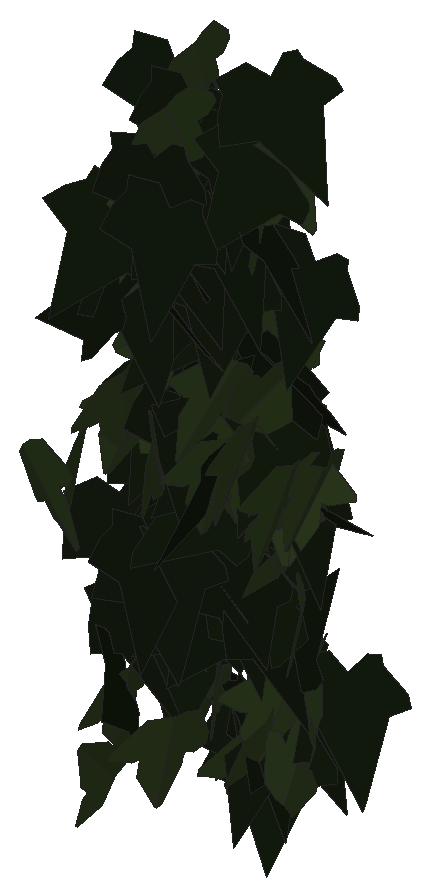
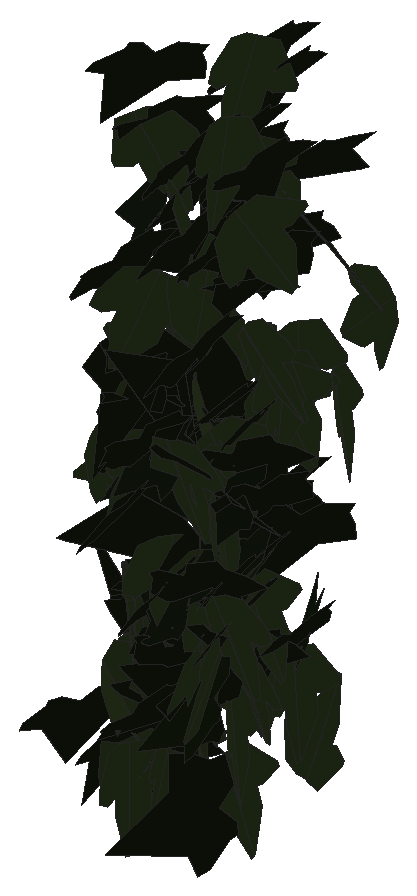
# SketchUp Ruby script. Lengths in inches.
U = 1.inch
M = Sketchup.active_model
def pt(a) = Geom::Point3d.new(a.map { |v| v * U })
def face(e, loops, mat)
  f = e.add_face(loops[0].map { |a| pt(a) })
  loops[1..].each { |l| e.add_face(l.map { |a| pt(a) }).erase! }
  f.material = f.back_material = mat if mat
  f
end
# faces: each face lists its corners as indices into pts; further lists are holes
def faces(e, pts, list, mat = nil) = list.each { |f| face(e, (f[0].is_a?(Array) ? f : [f]).map { |l| l.map { |i| pts[i] } }, mat) }
# xy, xz, yz: faces in a plane at the given z, y or x. An outline is a flat list of corners, or four numbers for a rectangle; further outlines are holes
def ring(l) = l.size == 4 ? [[l[0], l[1]], [l[2], l[1]], [l[2], l[3]], [l[0], l[3]]] : l.each_slice(2).to_a
def flat(e, list, mat, &to3) = list.each { |f| face(e, (f[0].is_a?(Array) ? f : [f]).map { |l| ring(l).map { |u, v| to3.(u, v) } }, mat) }
def xy(e, z, list, mat = nil) = flat(e, list, mat) { |x, y| [x, y, z] }
def xz(e, y, list, mat = nil) = flat(e, list, mat) { |x, z| [x, y, z] }
def yz(e, x, list, mat = nil) = flat(e, list, mat) { |y, z| [x, y, z] }
def lines(e, pts, list) = list.each { |a, b| e.add_line(pt(pts[a]), pt(pts[b])) }
# prism: a flat outline (further loops are holes) pulled along v
def prism(e, loops, v, mat = nil)
  f = face(e, loops, mat); d = Geom::Vector3d.new(v.map { |x| x * U })
  f.pushpull(f.normal.samedirection?(d) ? d.length : -d.length)
end
def box(e, o, s, mat = nil) = prism(e, [[o, [o[0] + s[0], o[1], o[2]], [o[0] + s[0], o[1] + s[1], o[2]], [o[0], o[1] + s[1], o[2]]]], [0, 0, s[2]], mat)
def at(x, y, z, deg = 0) = Geom::Transformation.translation(pt([x, y, z])) * Geom::Transformation.rotation(ORIGIN, Z_AXIS, deg.degrees)
def axes(o, x, y, z) = Geom::Transformation.new([*x, 0, *y, 0, *z, 0, *pt(o).to_a, 1])
def part(name) = M.definitions.add(name)
# library, detail: a bought-in or finely detailed component or shape, given as its bounding box
def library(name, o, s) = part(name).tap { |d| box(d.entities, o, s) }
def detail(e, o, s) = box(e.add_group.entities, o, s)
def put(e, d, t, mat = nil) = e.add_instance(d, t).tap { |i| i.material = mat if mat }
def group(e, t, mat = nil) = e.add_group.tap { |g| g.transformation = t; g.material = mat if mat }.entities
root = M.entities
M.materials.add("efeu1").color = [18, 25, 13]
M.materials.add("efeu2").color = [43, 57, 29]
c1 = part("ivyleaf_10")
p = [[0,0.5,-0.03],[-0.0625,2.02,-0.43],[-0.19,2.01,-0.46],[-0.54,1.05,-0.29],[-0.52,0.625,-0.18],[-0.83,0.76,-0.28],
  [-1.16,0.64,-0.33],[-1.15,0.33,-0.24],[-0.77,-0.39,0.02],[-0.3,-0.51,0.16],[0.04,-0.48,0.23],[-0.02,2.01,-0.4375],
  [-0.06,2.01,-0.43],[0.04,-0.49,0.23],[0.67,-0.49,0.14],[1.38,0.36,-0.2],[1.375,0.51,-0.24],[0.81,0.65,-0.19],
  [0.62,0.59,-0.15],[0.6,1.09,-0.28],[0.5,1.23,-0.31]]
faces(c1.entities,p,[[0,1,2,3,4,5,6,7,8,9,10],[11,12,0,13,14,15,16,17,18,19,20]],"efeu2")
c2 = part("ivyleaf_9")
p = [[1.54,2.16,1.25],[1.36,2.04,1.19],[-0.21,0.99,0.68],[-0.71,1.11,0.82],[-0.85,0.86,0.67],[-0.8,0.17,0.21],
  [-0.9,-0.01,0.1],[-0.67,-0.16,-0.02],[-0.08,-0.08,-0.05],[-0.03,-0.6,-0.4],[0.65,-0.88,-0.66],[0.83,-0.6,-0.49],
  [1.29,-0.42,-0.43],[1.8125,-0.07,-0.26],[1.21,0.44,0.15]]
faces(c2.entities,p,[[0,1,2,3,4,5,6,7,8,9,10,11,12,13,14]],"efeu1")
put(root,c1,axes([21.42,223.09,234.66],[0.162,-0.45556,-0.12737],[-0.01354,0.13011,-0.48258],[0.47284,0.1598,0.02982]))
put(root,c1,axes([21.47,223.21,235.97],[0.45383,-0.08336,-0.19259],[-0.1748,0.10376,-0.45681],[0.11612,0.48196,0.06503]))
put(root,c1,axes([21.52,222.74,240.73],[-0.16134,-0.38229,0.27896],[-0.05629,-0.27714,-0.41234],[0.46989,-0.16446,0.04639]))
put(root,c1,axes([21.4,222.91,235.22],[0.44303,-0.23126,-0.0156],[-0.01307,0.00866,-0.49975],[0.23141,0.44322,0.00163]))
put(root,c1,axes([21.46,221.16,237.97],[0.20397,-0.44652,-0.09496],[-0.01699,0.09651,-0.4903],[0.45619,0.20324,0.02419]))
put(root,c2,axes([21.33,222.99,241.68],[-0.10782,-0.48667,0.03903],[-0.0065,-0.03854,-0.49847],[0.48819,-0.10799,0.00199]))
put(root,c1,axes([21.48,222.62,235.85],[0.05393,-0.48608,0.10401],[0.00285,-0.10432,-0.48899],[0.49708,0.05333,-0.00848]))
put(root,c1,axes([21.42,221.75,233.52],[-0.04473,-0.33215,-0.37105],[-0.02937,-0.37013,0.33487],[-0.49713,0.05175,0.0136]))
put(root,c1,axes([21.51,221.875,234.64],[-0.00249,-0.49392,-0.07773],[0.01152,0.07765,-0.4938],[0.49986,-0.00425,0.011]))
put(root,c1,axes([21.52,223.01,233.81],[0.02957,-0.4962,0.05394],[-0.00482,-0.05432,-0.49702],[0.4991,0.02887,-0.00799]))
put(root,c1,axes([21.7,222.32,238.99],[0.3077,-0.16583,-0.35752],[-0.32173,0.15627,-0.34938],[0.22762,0.44506,-0.01054]))
put(root,c2,axes([21.26,222.3,235.39],[0.1524,-0.45433,-0.14269],[-0.00329,0.14882,-0.47733],[0.4762,0.14643,0.04237]))
put(root,c2,axes([21.54,222.94,237.9],[-0.3472,-0.35905,-0.02316],[0.01678,0.01599,-0.49946],[0.3594,-0.3476,0.00095]))
put(root,c2,axes([21.33,222.05,236.78],[-0.05664,-0.4023,-0.29145],[0.09276,0.27962,-0.40399],[0.48804,-0.09984,0.04296]))
put(root,c1,axes([21.54,223.25,235.35],[0.06205,-0.30518,-0.39118],[0.02748,0.39573,-0.30437],[0.49537,0.01627,0.06588]))
put(root,c1,axes([21.69,221.99,238.2],[-0.16252,-0.43116,0.19414],[-0.05936,-0.18505,-0.46069],[0.46911,-0.17279,0.00896]))
put(root,c2,axes([21.39,222.72,237.39],[0.00068,-0.44657,-0.2249],[0.06698,0.22295,-0.4425],[0.49549,-0.02953,0.06012]))
put(root,c1,axes([21.6,223.01,241.97],[-0.04509,-0.46727,-0.17213],[0.06125,0.16631,-0.46753],[0.49418,-0.06325,0.04224]))
put(root,c2,axes([21.26,223.68,233.76],[0.46894,-0.04796,0.16672],[0.16587,-0.0168,-0.47138],[0.05082,0.49741,0.00015]))
put(root,c1,axes([21.63,221.93,238.46],[-0.0639,-0.47515,-0.14196],[0.03474,0.13849,-0.47918],[0.49468,-0.0711,0.01532]))
put(root,c2,axes([21.75,223.53,236.5],[-0.4103,-0.28437,-0.02805],[0.02085,0.01915,-0.4992],[0.28499,-0.41081,-0.00386]))
put(root,c2,axes([21.45,222.77,236.49],[0.279,-0.33817,-0.24042],[-0.03835,0.26746,-0.42071],[0.41314,0.25319,0.1233]))
put(root,c2,axes([21.48,223.03,235.84],[0.11319,-0.48436,0.05084],[0.01191,-0.04943,-0.49741],[0.48687,0.11382,0.00035]))
put(root,c1,axes([21.77,223.03,235.92],[-0.08785,-0.49191,-0.01746],[0.00569,0.01672,-0.49969],[0.49219,-0.08799,0.00266]))
put(root,c2,axes([21.43,223.52,235.05],[0.41223,-0.28063,0.03616],[0.02669,-0.02504,-0.49866],[0.28169,0.41306,-0.00567]))
put(root,c1,axes([21.78,221.48,238.6],[-0.06652,-0.48285,-0.11149],[0.0163,0.1103,-0.48741],[0.49529,-0.06848,0.00106]))
put(root,c1,axes([21.79,222.87,237.08],[0.13997,-0.4719,-0.08784],[-0.01744,0.08644,-0.49216],[0.47969,0.14084,0.00774]))
put(root,c1,axes([21.82,222.875,237.83],[-0.12017,-0.44529,0.19308],[-0.02103,-0.19395,-0.46037],[0.48489,-0.11876,0.02788]))
put(root,c2,axes([22.1,221.02,239.98],[-0.36896,0.29037,0.17192],[-0.14342,0.09564,-0.46934],[-0.30545,-0.39565,0.01272]))
put(root,c2,axes([21.58,223.08,235.98],[0.04576,-0.44794,0.21739],[0.05491,-0.21244,-0.44928],[0.49486,0.06499,0.02975]))
put(root,c1,axes([21.68,222.75,237.7],[0.31352,0.38523,0.05747],[0.03252,0.04762,-0.49666],[-0.38813,0.31517,0.00481]))
put(root,c2,axes([21.63,221.74,234.6875],[-0.0113,-0.18597,0.46399],[0.03554,-0.46323,-0.1848],[0.49861,0.02881,0.02369]))
put(root,c1,axes([21.8,223.31,235.375],[-0.09842,0.45616,-0.17954],[-0.01552,-0.18593,-0.46389],[-0.48997,-0.08574,0.05075]))
put(root,c2,axes([21.8,222.66,235.18],[-0.22963,-0.42092,-0.14176],[0.05633,0.13069,-0.47932],[0.44056,-0.2361,-0.0126]))
put(root,c2,axes([21.93,221.29,240.81],[-0.2595,-0.39055,0.17357],[-0.03458,-0.18322,-0.46394],[0.42598,-0.25279,0.06808]))
put(root,c2,axes([21.8125,222.875,237.8],[-0.05662,-0.43271,0.24404],[-0.01462,-0.24406,-0.43614],[0.49657,-0.05653,0.01498]))
put(root,c2,axes([21.53,222.89,237.39],[0.36789,-0.17911,0.28736],[0.28472,-0.06605,-0.40568],[0.18329,0.46212,0.05339]))
put(root,c2,axes([21.59,222.74,236.25],[0.31209,-0.31312,0.23357],[0.16264,-0.16767,-0.44208],[0.35517,0.35192,-0.0028]))
put(root,c2,axes([22.28,223.18,237.62],[-0.4651,0.1003,0.1537],[-0.16048,-0.01909,-0.47316],[-0.08905,-0.48946,0.04995]))
put(root,c2,axes([21.54,223.33,234.87],[0.26945,-0.16012,0.38956],[0.34176,-0.18717,-0.31332],[0.24617,0.43512,0.00857]))
put(root,c2,axes([22.05,223.44,235.54],[-0.39421,-0.30689,-0.02043],[0.02036,0.0071,-0.49953],[0.3069,-0.39467,0.0069]))
put(root,c1,axes([22.06,223.32,237.83],[0.46354,-0.10321,-0.15646],[-0.14039,0.08538,-0.47223],[0.12419,0.48172,0.05018]))
put(root,c2,axes([21.81,222.45,238.43],[0.26422,-0.3478,-0.24336],[-0.02053,0.27584,-0.41652],[0.42399,0.2301,0.13148]))
put(root,c2,axes([21.9,222.57,241.67],[-0.0097,-0.49632,0.05973],[0.00706,-0.05987,-0.49635],[0.49986,-0.00878,0.00817]))
put(root,c2,axes([21.92,221.9,239.99],[0.04285,-0.36339,-0.34075],[0.01933,0.34297,-0.36332],[0.49779,0.01796,0.04344]))
put(root,c1,axes([21.95,223.07,234.23],[0.24182,-0.33251,0.28454],[0.22902,-0.18087,-0.406],[0.37293,0.32668,0.06483]))
put(root,c2,axes([22.33,222.28,237.85],[-0.41943,0.25092,-0.10543],[0.08583,-0.06185,-0.48868],[-0.25828,-0.42803,0.00881]))
put(root,c1,axes([22.18,222.15,235.93],[0.03203,-0.4986,0.0194],[-0.00168,-0.01955,-0.49961],[0.49897,0.03194,-0.00292]))
put(root,c1,axes([21.92,219.87,238.37],[-0.31494,0.19918,-0.33337],[0.27708,-0.18548,-0.37259],[-0.27209,-0.41943,0.00645]))
put(root,c1,axes([22.2,223.27,236.48],[-0.31951,-0.38451,-0.00816],[0.01625,-0.0029,-0.49973],[0.38426,-0.3196,0.01435]))
put(root,c2,axes([22.04,221.65,240.02],[-0.11955,-0.4542,-0.17148],[0.05718,0.1622,-0.46949],[0.48212,-0.13187,0.01316]))
put(root,c1,axes([21.97,222.98,234.72],[0.20651,-0.23119,0.3923],[0.289,-0.26635,-0.30909],[0.3519,0.35441,0.02362]))
put(root,c2,axes([22.37,223.03,235.51],[-0.01547,-0.09452,-0.49074],[-0.05993,-0.48708,0.0957],[-0.49615,0.06178,0.00374]))
put(root,c2,axes([22.01,223.15,239.18],[0.06323,-0.49592,0.00777],[0.00002,-0.00783,-0.49994],[0.49599,0.06323,-0.00098]))
put(root,c1,axes([22.34,221.69,240.8],[-0.29747,-0.27255,0.29534],[-0.06766,-0.32823,-0.37106],[0.39615,-0.26073,0.1584]))
put(root,c2,axes([22.07,222.19,238.1],[0.02234,-0.49726,0.04722],[0.01219,-0.04671,-0.49766],[0.49935,0.02339,0.01004]))
put(root,c2,axes([21.875,223.41,236.09],[0.1938,-0.3143,0.33713],[0.25838,-0.22877,-0.36181],[0.38168,0.31445,0.07375]))
put(root,c2,axes([22.11,221.62,236.62],[-0.027,-0.49436,0.06986],[0.00566,-0.07026,-0.49501],[0.49924,-0.02594,0.00939]))
put(root,c1,axes([22.28,222.56,238.28],[0.18808,-0.4428,0.13623],[0.03591,-0.13265,-0.48074],[0.46188,0.19062,-0.0181]))
put(root,c2,axes([22.36,222.23,239.5],[-0.32719,-0.33596,0.17342],[-0.03203,-0.20389,-0.45541],[0.37672,-0.30912,0.11191]))
put(root,c2,axes([22.32,222.68,237.5],[-0.23483,-0.32717,0.29634],[-0.04741,-0.31502,-0.38537],[0.43887,-0.20909,0.11693]))
put(root,c2,axes([22.21,221.67,236.59],[-0.16636,-0.40324,-0.24438],[0.09809,0.22387,-0.43619],[0.4612,-0.19307,0.00462]))
put(root,c1,axes([22.41,221.54,234.47],[-0.16861,-0.46925,0.03704],[-0.00513,-0.03752,-0.49856],[0.47068,-0.16851,0.00784]))
put(root,c1,axes([22.33,222.625,237.33],[0.38143,-0.32307,0.01158],[0.00448,-0.01262,-0.49982],[0.32325,0.3814,-0.00673]))
put(root,c2,axes([22.2,223.04,240.55],[0.02159,-0.49932,0.01473],[0.00105,-0.0147,-0.49978],[0.49953,0.02161,0.00041]))
put(root,c2,axes([22.52,222.46,237.01],[-0.40354,-0.2211,0.19563],[-0.08536,-0.2298,-0.43578],[0.28261,-0.38511,0.14772]))
put(root,c2,axes([22.29,222.51,235.57],[-0.11579,-0.37438,0.31053],[-0.00772,-0.31775,-0.38597],[0.48635,-0.09417,0.0678]))
put(root,c2,axes([22.22,223.46,236.12],[0.01098,-0.48222,0.13171],[0.01839,-0.13126,-0.48211],[0.49954,0.01544,0.01485]))
put(root,c2,axes([22.32,222.46,240.03],[-0.09351,-0.44748,0.20254],[-0.0305,-0.20049,-0.45703],[0.49023,-0.09783,0.0102]))
put(root,c1,axes([22.4,223.02,233.875],[0.07984,-0.44422,-0.21515],[0.07986,0.22671,-0.43844],[0.48708,0.03565,0.10715]))
put(root,c1,axes([22.41,221.56,242.11],[-0.15354,-0.42667,-0.21066],[0.09556,0.18919,-0.45285],[0.46615,-0.17932,0.02345]))
put(root,c2,axes([22.12,221.99,239.96],[0.05661,-0.18017,0.46296],[0.24382,-0.3959,-0.18389],[0.43284,0.24658,0.04304]))
put(root,c1,axes([22.47,221.14,238.18],[0.22506,-0.35692,-0.26825],[-0.01341,0.29487,-0.40358],[0.44628,0.18885,0.12315]))
put(root,c1,axes([22.33,222.29,237.83],[-0.43066,0.14503,-0.20857],[0.17682,-0.12363,-0.45105],[-0.18241,-0.46226,0.0552]))
put(root,c2,axes([22.375,223.71,234.62],[-0.14768,-0.45278,0.15225],[0.00242,-0.16006,-0.47368],[0.47769,-0.13917,0.04947]))
put(root,c2,axes([22.17,222.59,238.04],[0.05966,-0.10767,0.48461],[0.47529,0.15329,-0.02445],[-0.14331,0.46358,0.12064]))
put(root,c1,axes([22.4,222.59,239.15],[-0.03542,-0.36064,-0.34451],[0.03239,-0.34631,0.35919],[-0.49769,0.00313,0.0479]))
put(root,c1,axes([22.6,223.5,233.77],[-0.06793,-0.48401,-0.10543],[0.01343,0.10458,-0.48876],[0.49518,-0.06923,-0.0012]))
put(root,c2,axes([22.42,221.27,241.68],[0.00056,-0.49968,-0.01774],[0.00323,0.01774,-0.49967],[0.49999,0.00045,0.00325]))
put(root,c2,axes([22.32,222.96,237.89],[0.45104,-0.21578,0.00117],[0.00104,-0.00053,-0.5],[0.21578,0.45104,-0.00003]))
put(root,c1,axes([22.69,222.77,233.83],[-0.20021,-0.45679,0.03543],[-0.00656,-0.03581,-0.49867],[0.45812,-0.20014,0.00834]))
put(root,c2,axes([22.49,222.66,241.32],[0.00436,-0.49268,0.08515],[0.00196,-0.08513,-0.4927],[0.49998,0.00463,0.00119]))
put(root,c2,axes([22.42,223.25,233.88],[0.13552,-0.46598,0.12038],[0.02819,-0.11716,-0.48526],[0.48046,0.13831,-0.00549]))
put(root,c2,axes([22.98,222.93,235.625],[-0.41003,-0.01845,0.28555],[-0.24723,-0.22838,-0.36976],[0.14407,-0.44441,0.17816]))
put(root,c2,axes([22.3125,223.02,236.86],[0.42334,-0.05675,0.25992],[0.26398,0.02889,-0.42365],[0.03306,0.49593,0.05443]))
put(root,c1,axes([22.75,223.47,233.99],[0.01329,-0.49693,-0.05366],[0.00313,0.05376,-0.49709],[0.49981,0.01288,0.00454]))
put(root,c2,axes([22.69,223.18,237.8125],[-0.21508,-0.44975,0.03821],[-0.01308,-0.03609,-0.49852],[0.45119,-0.21545,0.00376]))
put(root,c2,axes([22.58,221.57,240.88],[0.03873,-0.44296,-0.22867],[-0.0182,0.22795,-0.44465],[0.49817,0.04277,0.00153]))
put(root,c2,axes([22.53,223,233.96],[0.01206,-0.31777,0.38585],[0.08535,-0.37898,-0.31478],[0.49251,0.07346,0.04511]))
put(root,c1,axes([22.76,222.91,236.0625],[-0.00585,-0.46562,-0.18211],[0.03678,0.18123,-0.46455],[0.49861,-0.01884,0.03213]))
put(root,c2,axes([22.99,222.78,238.69],[0.16494,0.10145,-0.46098],[-0.38257,-0.25728,-0.19351],[-0.27646,0.41655,-0.00725]))
put(root,c2,axes([22.59,222.54,236.14],[0.05196,-0.48821,-0.09459],[-0.00709,0.09437,-0.49096],[0.49724,0.05236,0.00288]))
put(root,c1,axes([22.85,221.93,238.84],[-0.07036,-0.4031,0.28734],[-0.00575,-0.28954,-0.40759],[0.49499,-0.06066,0.03611]))
put(root,c2,axes([22.72,222.14,240.13],[-0.17256,-0.46099,-0.08783],[0.02149,0.08572,-0.49213],[0.46879,-0.17362,-0.00977]))
put(root,c2,axes([22.73,223.04,233.81],[-0.22931,-0.4162,-0.15556],[0.06556,0.14144,-0.47507],[0.43945,-0.23827,-0.0103]))
put(root,c1,axes([22.89,221.8125,237.97],[-0.12038,-0.48031,0.06937],[0.00492,-0.07267,-0.49467],[0.48527,-0.11841,0.02223]))
put(root,c2,axes([22.66,223.43,234.24],[0.12808,-0.42708,-0.22627],[-0.03906,0.22417,-0.44522],[0.48174,0.13172,0.02406]))
put(root,c1,axes([22.87,222.42,240.62],[0.36772,-0.33729,-0.03191],[-0.02365,0.02142,-0.49898],[0.33797,0.36848,-0.0002]))
put(root,c2,axes([22.875,221.97,237.81],[-0.17867,0.00887,-0.4669],[0.30861,-0.37295,-0.12517],[-0.35048,-0.33291,0.12779]))
put(root,c2,axes([22.83,222.72,234.28],[-0.37046,-0.24949,-0.22476],[0.25393,0.01085,-0.43058],[0.21973,-0.43317,0.11866]))
put(root,c2,axes([22.71,222.21,240.67],[0.11842,-0.47875,-0.08232],[-0.01737,0.0805,-0.49317],[0.48546,0.11966,0.00243]))
put(root,c1,axes([22.91,223.4,234.76],[0.17003,-0.43967,0.16668],[0.04421,-0.1615,-0.47113],[0.46812,0.17495,-0.01604]))
put(root,c2,axes([22.93,222.91,238.04],[-0.39524,-0.28045,-0.12304],[0.11328,0.05275,-0.48413],[0.28453,-0.41057,0.02184]))
put(root,c1,axes([22.86,222.84,239.5],[-0.37807,-0.27424,-0.17847],[0.17516,0.06072,-0.46436],[0.27637,-0.41365,0.05016]))
put(root,c1,axes([23,222.47,234.27],[-0.02703,-0.45176,-0.21257],[0.01803,0.21186,-0.45254],[0.49894,-0.03213,0.00484]))
put(root,c2,axes([22.75,222.63,235.66],[0.21542,-0.43936,-0.10275],[-0.01279,0.10787,-0.48806],[0.45103,0.2129,0.03523]))
put(root,c1,axes([23.01,222.06,238.09],[0.13079,-0.46534,0.12789],[0.0348,-0.12307,-0.48337],[0.48133,0.13534,0.00019]))
put(root,c2,axes([22.82,223.34,236.97],[0.08733,-0.49231,0.00296],[0.01018,-0.0012,-0.49989],[0.49221,0.08737,0.00981]))
put(root,c2,axes([22.77,221.14,239.98],[0.44231,-0.15932,-0.17024],[0.15964,-0.05915,0.47012],[-0.16994,-0.47023,-0.00146]))
put(root,c1,axes([23.12,222.65,234.71],[-0.25172,-0.38664,0.19273],[-0.02721,-0.20843,-0.45367],[0.43116,-0.23888,0.0839]))
put(root,c1,axes([22.91,222.45,238.28],[-0.05239,-0.38455,0.31524],[0.08825,0.30476,0.38643],[-0.48935,0.09613,0.03594]))
put(root,c1,axes([23.21,222.45,241.29],[0.41615,0.07069,-0.26799],[-0.27714,0.10037,-0.40388],[-0.00331,0.48469,0.12272]))
put(root,c1,axes([23.125,222.875,235.64],[0.26561,-0.37791,-0.1914],[-0.05921,0.19057,-0.45845],[0.41946,0.2662,0.05648]))
put(root,c1,axes([23.0625,222.64,237.22],[-0.11487,-0.36628,-0.32038],[0.11533,0.29932,-0.38355],[0.47276,-0.16201,0.01572]))
put(root,c2,axes([23.05,222.79,238.54],[0.44076,0.05916,-0.22855],[-0.22938,-0.00721,-0.44422],[-0.05585,0.49644,0.02078]))
put(root,c2,axes([23.14,222.45,241.47],[-0.30139,-0.37325,0.1409],[-0.04201,-0.14591,-0.47639],[0.39674,-0.29899,0.05659]))
put(root,c1,axes([23.02,222.91,237.29],[0.39065,0.312,-0.00661],[-0.00514,-0.00416,-0.49996],[-0.31203,0.39069,-0.00004]))
put(root,c2,axes([22.98,222.85,235],[-0.21176,0.2508,0.37717],[0.2234,-0.30436,0.32781],[0.39402,0.30735,0.01685]))
put(root,c2,axes([23.09,220.68,241.54],[-0.07289,-0.49267,0.04428],[-0.00043,-0.0447,-0.498],[0.49466,-0.07264,0.00609]))
put(root,c2,axes([23.05,222.53,242.35],[-0.01638,-0.39729,-0.30314],[0.11636,0.29194,-0.38889],[0.486,-0.08329,0.08289]))
put(root,c2,axes([22.97,222.41,240.59],[0.28183,-0.3956,0.11865],[0.06745,-0.09762,-0.48572],[0.40746,0.28978,-0.00166]))
put(root,c1,axes([23.33,222.99,237.43],[0.017,-0.47208,0.16386],[-0.00035,-0.16396,-0.47235],[0.49971,0.01595,-0.0059]))
put(root,c2,axes([23.19,223.06,239.88],[-0.09975,-0.48428,0.07429],[-0.00101,-0.07561,-0.49425],[0.48995,-0.09875,0.01411]))
put(root,c1,axes([23.32,222.37,237.52],[0.06509,-0.46542,0.17073],[0.04783,-0.1655,-0.46939],[0.49343,0.07744,0.02298]))
put(root,c2,axes([23.17,223.69,234.47],[-0.0906,-0.46271,-0.16642],[0.07034,0.15528,-0.47004],[0.48667,-0.10858,0.03696]))
put(root,c1,axes([23.36,222.4,233.8],[0.00381,0.31736,-0.38636],[0.01931,0.38599,0.31724],[0.49961,-0.01734,-0.00932]))
